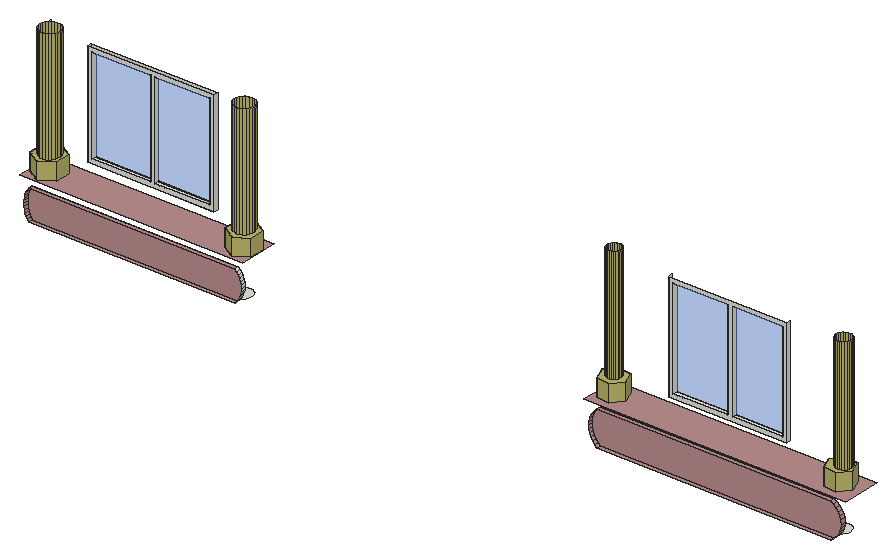
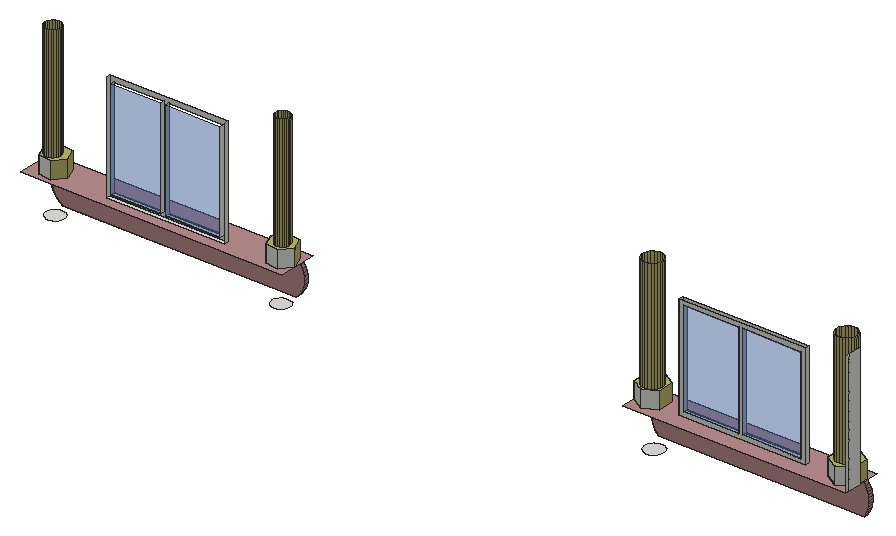
# SketchUp Ruby script. Lengths in inches.
U = 1.inch
M = Sketchup.active_model
def pt(a) = Geom::Point3d.new(a.map { |v| v * U })
def face(e, loops, mat)
  f = e.add_face(loops[0].map { |a| pt(a) })
  loops[1..].each { |l| e.add_face(l.map { |a| pt(a) }).erase! }
  f.material = f.back_material = mat if mat
  f
end
# faces: each face lists its corners as indices into pts; further lists are holes
def faces(e, pts, list, mat = nil) = list.each { |f| face(e, (f[0].is_a?(Array) ? f : [f]).map { |l| l.map { |i| pts[i] } }, mat) }
# xy, xz, yz: faces in a plane at the given z, y or x. An outline is a flat list of corners, or four numbers for a rectangle; further outlines are holes
def ring(l) = l.size == 4 ? [[l[0], l[1]], [l[2], l[1]], [l[2], l[3]], [l[0], l[3]]] : l.each_slice(2).to_a
def flat(e, list, mat, &to3) = list.each { |f| face(e, (f[0].is_a?(Array) ? f : [f]).map { |l| ring(l).map { |u, v| to3.(u, v) } }, mat) }
def xy(e, z, list, mat = nil) = flat(e, list, mat) { |x, y| [x, y, z] }
def xz(e, y, list, mat = nil) = flat(e, list, mat) { |x, z| [x, y, z] }
def yz(e, x, list, mat = nil) = flat(e, list, mat) { |y, z| [x, y, z] }
def lines(e, pts, list) = list.each { |a, b| e.add_line(pt(pts[a]), pt(pts[b])) }
# prism: a flat outline (further loops are holes) pulled along v
def prism(e, loops, v, mat = nil)
  f = face(e, loops, mat); d = Geom::Vector3d.new(v.map { |x| x * U })
  f.pushpull(f.normal.samedirection?(d) ? d.length : -d.length)
end
def box(e, o, s, mat = nil) = prism(e, [[o, [o[0] + s[0], o[1], o[2]], [o[0] + s[0], o[1] + s[1], o[2]], [o[0], o[1] + s[1], o[2]]]], [0, 0, s[2]], mat)
def at(x, y, z, deg = 0) = Geom::Transformation.translation(pt([x, y, z])) * Geom::Transformation.rotation(ORIGIN, Z_AXIS, deg.degrees)
def axes(o, x, y, z) = Geom::Transformation.new([*x, 0, *y, 0, *z, 0, *pt(o).to_a, 1])
def part(name) = M.definitions.add(name)
# library, detail: a bought-in or finely detailed component or shape, given as its bounding box
def library(name, o, s) = part(name).tap { |d| box(d.entities, o, s) }
def detail(e, o, s) = box(e.add_group.entities, o, s)
def put(e, d, t, mat = nil) = e.add_instance(d, t).tap { |i| i.material = mat if mat }
def group(e, t, mat = nil) = e.add_group.tap { |g| g.transformation = t; g.material = mat if mat }.entities
root = M.entities
M.materials.add("[0057_DarkKhaki]").color = [189, 183, 107]
M.materials.add("[0119_RosyBrown]").color = [188, 143, 143]
M.materials.add("[Translucent Glass Blue]").color = [100, 149, 237]
M.materials["[Translucent Glass Blue]"].alpha = 0.5
xy(root,364,[[551.49,97.26,553.12,97.47,554.64,98.1,555.95,99.11,556.95,100.41,557.58,101.9375,557.8,103.57,557.58,105.2,556.95,106.73,555.95,108.03,554.64,109.04,553.12,109.67,551.49,109.88,549.85,109.67,548.33,109.04,547.02,108.03,546.02,106.73,545.39,105.2,545.17,103.57,545.39,101.9375,546.02,100.41,547.02,99.11,548.33,98.1,549.85,97.47],[711.11,97.26,712.74,97.47,714.27,98.1,715.57,99.11,716.58,100.41,717.21,101.9375,717.42,103.57,717.21,105.2,716.58,106.73,715.57,108.03,714.27,109.04,712.74,109.67,711.11,109.88,709.48,109.67,707.95,109.04,706.65,108.03,705.64,106.73,705.01,105.2,704.8,103.57,705.01,101.9375,705.64,100.41,706.65,99.11,707.95,98.1,709.48,97.47]])
xy(root,364,[[549.67,89.37,714.61,92.37]],"[0119_RosyBrown]")
xy(root,364.25,[[287.6,96.4,289.34,96.48,291.01,97.01,292.47,97.96,293.65,99.25,294.45,100.8,294.82,102.51,294.74,104.25,294.21,105.91,293.26,107.38,291.97,108.56,290.42,109.36,288.71,109.73,286.97,109.65,285.31,109.11,283.84,108.17,282.66,106.88,281.86,105.33,281.49,103.62,281.58,101.88,282.11,100.22,283.05,98.75,284.34,97.57,285.89,96.77]])
xy(root,366,[[148.36,89.37,293.68,92.37]],"[0119_RosyBrown]")
xy(root,387.6875,[[148.36,89.37,293.68,92.37]],"[0119_RosyBrown]")
xy(root,388.75,[[549.67,89.37,714.61,92.37]],"[0119_RosyBrown]")
xy(root,391.75,[[540.59,104.78,540.59,105.17,540.49,105.04]])
xy(root,391.75,[[[540.59,89.37,725.37,89.37,725.37,116.37,540.59,116.37,540.59,105.17,546.55,112.6,556.13,111.125,559.64,102.1,553.58,94.54,544,96.01,540.59,104.78],[713.95,94.54,704.38,96.01,700.87,105.04,706.93,112.6,716.5,111.125,720.02,102.1]]],"[0119_RosyBrown]")
xy(root,393.6875,[[152.83,91.15,143.52,96.53,143.52,107.28,152.83,112.65,162.14,107.28,162.14,96.53],[290.08,91.15,280.77,96.53,280.77,107.28,290.08,112.65,299.39,107.28,299.39,96.53]])
xy(root,393.6875,[[[142.36,89.37,299.68,116.37],[290.08,91.15,280.77,96.53,280.77,107.28,290.08,112.65,299.39,107.28,299.39,96.53],[152.83,91.15,143.52,96.53,143.52,107.28,152.83,112.65,162.14,107.28,162.14,96.53]]],"[0119_RosyBrown]")
xy(root,397.08,[[581.28,113.37,664.4,116.37]])
xy(root,400.08,[[584.28,113.37,622.84,116.37],[626.17,113.37,661.4,116.37]])
xy(root,401.45,[[170.78,113.37,260.03,116.37]])
xy(root,403.75,[[711.84,99.06,710.41,99.24,709.09,99.79,707.95,100.67,707.07,101.81,706.53,103.13,706.34,104.56,706.53,105.98,707.07,107.31,707.95,108.44,709.09,109.32,710.41,109.87,711.84,110.06,713.26,109.87,714.59,109.32,715.73,108.44,716.6,107.31,717.15,105.98,717.34,104.56,717.15,103.13,716.6,101.81,715.73,100.67,714.59,99.79,713.26,99.24]])
xy(root,403.75,[[[553.58,94.54,559.64,102.1,556.13,111.125,546.55,112.6,540.59,105.17,540.59,104.78,544,96.01],[549.01,99.72,547.78,100.05,546.67,100.68,545.77,101.58,545.13,102.68,544.8,103.91,544.8,105.19,545.13,106.41,545.76,107.52,546.66,108.42,547.76,109.06,548.99,109.39,550.26,109.39,551.49,109.0625,552.6,108.43,553.5,107.53,554.14,106.43,554.47,105.2,554.47,103.93,554.14,102.7,553.51,101.59,552.61,100.69,551.51,100.05,550.28,99.72]],[[713.95,94.54,720.02,102.1,716.5,111.125,706.93,112.6,700.87,105.04,704.38,96.01],[711.84,99.06,710.41,99.24,709.09,99.79,707.95,100.67,707.07,101.81,706.53,103.13,706.34,104.56,706.53,105.98,707.07,107.31,707.95,108.44,709.09,109.32,710.41,109.87,711.84,110.06,713.26,109.87,714.59,109.32,715.73,108.44,716.6,107.31,717.15,105.98,717.34,104.56,717.15,103.13,716.6,101.81,715.73,100.67,714.59,99.79,713.26,99.24]]],"[0057_DarkKhaki]")
xy(root,404.45,[[173.78,113.37,215.4,116.37],[217.84,113.37,257.03,116.37]])
xy(root,405.6875,[[153.73,94.92,151.91,95.02,150.17,95.59,148.64,96.6,147.43,97.96,146.6,99.59,146.23,101.38,146.33,103.2,146.91,104.94,147.91,106.47,149.27,107.69,150.9,108.51,152.69,108.88,154.52,108.78,156.25,108.21,157.78,107.2,159,105.84,159.82,104.21,160.19,102.42,160.09,100.6,159.52,98.86,158.52,97.33,157.15,96.12,155.52,95.29],[289.98,96.17,288.16,96.27,286.42,96.84,284.89,97.85,283.68,99.21,282.85,100.84,282.48,102.63,282.58,104.45,283.16,106.19,284.16,107.72,285.52,108.94,287.15,109.76,288.94,110.13,290.77,110.03,292.5,109.46,294.03,108.45,295.25,107.09,296.07,105.46,296.44,103.67,296.34,101.85,295.77,100.11,294.77,98.58,293.4,97.37,291.77,96.54]])
xy(root,405.6875,[[[152.83,91.15,162.14,96.53,162.14,107.28,152.83,112.65,143.52,107.28,143.52,96.53],[153.73,94.92,151.91,95.02,150.17,95.59,148.64,96.6,147.43,97.96,146.6,99.59,146.23,101.38,146.33,103.2,146.91,104.94,147.91,106.47,149.27,107.69,150.9,108.51,152.69,108.88,154.52,108.78,156.25,108.21,157.78,107.2,159,105.84,159.82,104.21,160.19,102.42,160.09,100.6,159.52,98.86,158.52,97.33,157.15,96.12,155.52,95.29]],[[290.08,91.15,299.39,96.53,299.39,107.28,290.08,112.65,280.77,107.28,280.77,96.53],[289.98,96.17,288.16,96.27,286.42,96.84,284.89,97.85,283.68,99.21,282.85,100.84,282.48,102.63,282.58,104.45,283.16,106.19,284.16,107.72,285.52,108.94,287.15,109.76,288.94,110.13,290.77,110.03,292.5,109.46,294.03,108.45,295.25,107.09,296.07,105.46,296.44,103.67,296.34,101.85,295.77,100.11,294.77,98.58,293.4,97.37,291.77,96.54]]],"[0057_DarkKhaki]")
xz(root,92.37,[[549.67,364,714.61,364,716.81,365.33,718.71,367.04,720.27,369.07,721.42,371.36,722.13,373.82,722.37,376.375,722.13,378.93,721.42,381.39,720.27,383.68,718.71,385.71,716.81,387.42,714.61,388.75,549.67,388.75,547.9,387.16,546.4,385.32,545.19,383.27,544.3125,381.0625,543.77,378.75,543.59,376.375,543.77,374,544.3125,371.6875,545.19,369.48,546.4,367.43,547.9,365.59],[148.36,366,293.68,366,295.15,367.43,296.41,369.0625,297.41,370.86,298.14,372.78,298.59,374.79,298.74,376.84,298.59,378.9,298.14,380.9,297.41,382.83,296.41,384.625,295.15,386.26,293.68,387.6875,148.36,387.6875,147.34,386.06,146.48,384.33,145.81,382.53,145.32,380.67,145.03,378.77,144.93,376.84,145.03,374.92,145.32,373.02,145.81,371.16,146.48,369.35,147.34,367.63]],"[0119_RosyBrown]")
xz(root,99.72,[[549.01,403.75,550.28,484.5]],"[0057_DarkKhaki]")
xz(root,109.39,[[548.99,403.75,550.26,484.5]],"[0057_DarkKhaki]")
xz(root,113.37,[[[581.28,397.08,664.4,473.26],[584.28,400.08,622.84,470.26],[626.17,400.08,661.4,470.26]],[[170.78,401.45,260.03,475.13],[173.78,404.45,215.4,472.13],[217.84,404.45,257.03,472.13]]])
xz(root,116.37,[[[170.78,401.45,260.03,475.13],[173.78,404.45,215.4,472.13],[217.84,404.45,257.03,472.13]]])
xz(root,116.37,[[584.28,400.08,622.84,470.26],[626.17,400.08,661.4,470.26],[173.78,404.45,215.4,472.13],[217.84,404.45,257.03,472.13]],"[Translucent Glass Blue]")
yz(root,142.36,[[104.37,393.6875,113.37,480],[113.37,393.6875,116.37,480]])
yz(root,143.52,[[96.53,393.6875,107.28,405.6875]],"[0057_DarkKhaki]")
yz(root,162.14,[[96.53,393.6875,107.28,405.6875]],"[0057_DarkKhaki]")
yz(root,170.78,[[113.37,401.45,116.37,475.13]])
yz(root,173.78,[[113.37,404.45,116.37,472.13]])
yz(root,215.4,[[113.37,404.45,116.37,472.13]])
yz(root,217.84,[[113.37,404.45,116.37,472.13]])
yz(root,257.03,[[113.37,404.45,116.37,472.13]])
yz(root,260.03,[[113.37,401.45,116.37,475.13]])
yz(root,280.77,[[96.53,393.6875,107.28,405.6875]],"[0057_DarkKhaki]")
yz(root,299.39,[[96.53,393.6875,107.28,405.6875]],"[0057_DarkKhaki]")
yz(root,540.59,[[104.78,391.75,105.17,403.75]])
yz(root,544.8,[[103.91,403.75,105.19,484.5]],"[0057_DarkKhaki]")
yz(root,554.47,[[103.93,403.75,105.2,484.5]],"[0057_DarkKhaki]")
yz(root,581.28,[[113.37,397.08,116.37,473.26]])
yz(root,584.28,[[113.37,400.08,116.37,470.26]])
yz(root,622.84,[[113.37,400.08,116.37,470.26]])
yz(root,626.17,[[113.37,400.08,116.37,470.26]])
yz(root,661.4,[[113.37,400.08,116.37,470.26]])
yz(root,664.4,[[113.37,397.08,116.37,473.26]])
p = [[549.67,92.37,364],[547.9,92.37,365.59],[547.9,89.37,365.59],[549.67,89.37,364],[716.81,92.37,365.33],[714.61,92.37,364],
  [714.61,89.37,364],[716.81,89.37,365.33],[718.71,92.37,367.04],[718.71,89.37,367.04],[546.4,92.37,367.43],[546.4,89.37,367.43],
  [148.36,92.37,366],[147.34,92.37,367.63],[147.34,89.37,367.63],[148.36,89.37,366],[295.15,92.37,367.43],[293.68,92.37,366],
  [293.68,89.37,366],[295.15,89.37,367.43],[720.27,92.37,369.07],[720.27,89.37,369.07],[296.41,92.37,369.0625],[296.41,89.37,369.0625],
  [545.19,92.37,369.48],[545.19,89.37,369.48],[146.48,92.37,369.35],[146.48,89.37,369.35],[297.41,92.37,370.86],[297.41,89.37,370.86],
  [721.42,92.37,371.36],[721.42,89.37,371.36],[145.81,92.37,371.16],[145.81,89.37,371.16],[544.3125,92.37,371.6875],[544.3125,89.37,371.6875],
  [298.14,92.37,372.78],[298.14,89.37,372.78],[145.32,92.37,373.02],[145.32,89.37,373.02],[722.13,92.37,373.82],[722.13,89.37,373.82],
  [543.77,92.37,374],[543.77,89.37,374],[298.59,92.37,374.79],[298.59,89.37,374.79],[145.03,92.37,374.92],[145.03,89.37,374.92],
  [722.37,92.37,376.375],[722.37,89.37,376.375],[543.59,92.37,376.375],[543.59,89.37,376.375],[298.74,92.37,376.84],[298.74,89.37,376.84],
  [144.93,92.37,376.84],[144.93,89.37,376.84],[543.77,92.37,378.75],[543.77,89.37,378.75],[722.13,92.37,378.93],[722.13,89.37,378.93],
  [145.03,92.37,378.77],[145.03,89.37,378.77],[298.59,92.37,378.9],[298.59,89.37,378.9],[544.3125,92.37,381.0625],[544.3125,89.37,381.0625],
  [145.32,92.37,380.67],[145.32,89.37,380.67],[298.14,92.37,380.9],[298.14,89.37,380.9],[721.42,92.37,381.39],[721.42,89.37,381.39],
  [145.81,92.37,382.53],[145.81,89.37,382.53],[297.41,92.37,382.83],[297.41,89.37,382.83],[545.19,92.37,383.27],[545.19,89.37,383.27],
  [720.27,92.37,383.68],[720.27,89.37,383.68],[146.48,92.37,384.33],[146.48,89.37,384.33],[296.41,92.37,384.625],[296.41,89.37,384.625],
  [546.4,92.37,385.32],[546.4,89.37,385.32],[718.71,92.37,385.71],[718.71,89.37,385.71],[147.34,92.37,386.06],[147.34,89.37,386.06],
  [295.15,92.37,386.26],[295.15,89.37,386.26],[547.9,92.37,387.16],[547.9,89.37,387.16],[716.81,92.37,387.42],[716.81,89.37,387.42],
  [148.36,92.37,387.6875],[148.36,89.37,387.6875],[293.68,92.37,387.6875],[293.68,89.37,387.6875],[549.67,92.37,388.75],[549.67,89.37,388.75],
  [714.61,92.37,388.75],[714.61,89.37,388.75],[544,96.01,391.75],[553.58,94.54,391.75],[553.58,94.54,403.75],[544,96.01,403.75],
  [559.64,102.1,391.75],[559.64,102.1,403.75],[704.38,96.01,391.75],[713.95,94.54,391.75],[713.95,94.54,403.75],[704.38,96.01,403.75],
  [720.02,102.1,391.75],[720.02,102.1,403.75],[540.59,104.78,391.75],[540.59,104.78,403.75],[700.87,105.04,391.75],[700.87,105.04,403.75],
  [556.13,111.125,391.75],[556.13,111.125,403.75],[716.5,111.125,391.75],[716.5,111.125,403.75],[706.93,112.6,391.75],[706.93,112.6,403.75],
  [546.55,112.6,391.75],[540.59,105.17,391.75],[540.59,105.17,403.75],[546.55,112.6,403.75],[143.52,96.53,393.6875],[152.83,91.15,393.6875],
  [152.83,91.15,405.6875],[143.52,96.53,405.6875],[162.14,96.53,393.6875],[162.14,96.53,405.6875],[280.77,96.53,393.6875],[290.08,91.15,393.6875],
  [290.08,91.15,405.6875],[280.77,96.53,405.6875],[299.39,96.53,393.6875],[299.39,96.53,405.6875],[152.83,112.65,393.6875],[143.52,107.28,393.6875],
  [143.52,107.28,405.6875],[152.83,112.65,405.6875],[162.14,107.28,393.6875],[162.14,107.28,405.6875],[290.08,112.65,393.6875],[280.77,107.28,393.6875],
  [280.77,107.28,405.6875],[290.08,112.65,405.6875],[299.39,107.28,393.6875],[299.39,107.28,405.6875],[710.41,99.24,403.75],[711.84,99.06,403.75],
  [711.84,99.06,484.5],[710.41,99.24,484.5],[713.26,99.24,403.75],[713.26,99.24,484.5],[709.09,99.79,403.75],[709.09,99.79,484.5],
  [714.59,99.79,403.75],[714.59,99.79,484.5],[547.78,100.05,403.75],[549.01,99.72,403.75],[549.01,99.72,484.5],[547.78,100.05,484.5],
  [550.28,99.72,403.75],[551.51,100.05,403.75],[551.51,100.05,484.5],[550.28,99.72,484.5],[707.95,100.67,403.75],[707.95,100.67,484.5],
  [715.73,100.67,403.75],[715.73,100.67,484.5],[546.67,100.68,403.75],[546.67,100.68,484.5],[552.61,100.69,403.75],[552.61,100.69,484.5],
  [545.77,101.58,403.75],[545.77,101.58,484.5],[553.51,101.59,403.75],[553.51,101.59,484.5],[707.07,101.81,403.75],[707.07,101.81,484.5],
  [716.6,101.81,403.75],[716.6,101.81,484.5],[545.13,102.68,403.75],[545.13,102.68,484.5],[554.14,102.7,403.75],[554.14,102.7,484.5],
  [706.53,103.13,403.75],[706.53,103.13,484.5],[717.15,103.13,403.75],[717.15,103.13,484.5],[544.8,103.91,403.75],[544.8,103.91,484.5],
  [554.47,103.93,403.75],[554.47,103.93,484.5],[706.34,104.56,403.75],[706.34,104.56,484.5],[717.34,104.56,403.75],[717.34,104.56,484.5],
  [706.53,105.98,403.75],[706.53,105.98,484.5],[717.15,105.98,403.75],[717.15,105.98,484.5],[545.13,106.41,403.75],[544.8,105.19,403.75],
  [544.8,105.19,484.5],[545.13,106.41,484.5],[554.47,105.2,403.75],[554.14,106.43,403.75],[554.14,106.43,484.5],[554.47,105.2,484.5],
  [707.07,107.31,403.75],[707.07,107.31,484.5],[716.6,107.31,403.75],[716.6,107.31,484.5],[545.76,107.52,403.75],[545.76,107.52,484.5],
  [553.5,107.53,403.75],[553.5,107.53,484.5],[707.95,108.44,403.75],[707.95,108.44,484.5],[715.73,108.44,403.75],[715.73,108.44,484.5],
  [546.66,108.42,403.75],[546.66,108.42,484.5],[552.6,108.43,403.75],[552.6,108.43,484.5],[547.76,109.06,403.75],[547.76,109.06,484.5],
  [551.49,109.0625,403.75],[551.49,109.0625,484.5],[709.09,109.32,403.75],[709.09,109.32,484.5],[714.59,109.32,403.75],[714.59,109.32,484.5],
  [548.99,109.39,403.75],[548.99,109.39,484.5],[550.26,109.39,403.75],[550.26,109.39,484.5],[710.41,109.87,403.75],[710.41,109.87,484.5],
  [713.26,109.87,403.75],[713.26,109.87,484.5],[711.84,110.06,403.75],[711.84,110.06,484.5],[151.91,95.02,405.6875],[153.73,94.92,405.6875],
  [153.73,94.92,485.25],[151.91,95.02,485.25],[155.52,95.29,405.6875],[155.52,95.29,485.25],[150.17,95.59,405.6875],[150.17,95.59,485.25],
  [157.15,96.12,405.6875],[157.15,96.12,485.25],[148.64,96.6,405.6875],[148.64,96.6,485.25],[158.52,97.33,405.6875],[158.52,97.33,485.25],
  [288.16,96.27,405.6875],[289.98,96.17,405.6875],[289.98,96.17,485.25],[288.16,96.27,485.25],[291.77,96.54,405.6875],[291.77,96.54,485.25],
  [286.42,96.84,405.6875],[286.42,96.84,485.25],[293.4,97.37,405.6875],[293.4,97.37,485.25],[147.43,97.96,405.6875],[147.43,97.96,485.25],
  [284.89,97.85,405.6875],[284.89,97.85,485.25],[159.52,98.86,405.6875],[159.52,98.86,485.25],[294.77,98.58,405.6875],[294.77,98.58,485.25],
  [283.68,99.21,405.6875],[283.68,99.21,485.25],[146.6,99.59,405.6875],[146.6,99.59,485.25],[295.77,100.11,405.6875],[295.77,100.11,485.25],
  [160.09,100.6,405.6875],[160.09,100.6,485.25],[282.85,100.84,405.6875],[282.85,100.84,485.25],[146.23,101.38,405.6875],[146.23,101.38,485.25],
  [296.34,101.85,405.6875],[296.34,101.85,485.25],[160.19,102.42,405.6875],[160.19,102.42,485.25],[282.48,102.63,405.6875],[282.48,102.63,485.25],
  [146.33,103.2,405.6875],[146.33,103.2,485.25],[296.44,103.67,405.6875],[296.44,103.67,485.25],[159.82,104.21,405.6875],[159.82,104.21,485.25],
  [282.58,104.45,405.6875],[282.58,104.45,485.25],[146.91,104.94,405.6875],[146.91,104.94,485.25],[296.07,105.46,405.6875],[296.07,105.46,485.25],
  [159,105.84,405.6875],[159,105.84,485.25],[283.16,106.19,405.6875],[283.16,106.19,485.25],[147.91,106.47,405.6875],[147.91,106.47,485.25],
  [295.25,107.09,405.6875],[295.25,107.09,485.25],[157.78,107.2,405.6875],[157.78,107.2,485.25],[284.16,107.72,405.6875],[284.16,107.72,485.25],
  [149.27,107.69,405.6875],[149.27,107.69,485.25],[294.03,108.45,405.6875],[294.03,108.45,485.25],[156.25,108.21,405.6875],[156.25,108.21,485.25],
  [150.9,108.51,405.6875],[150.9,108.51,485.25],[285.52,108.94,405.6875],[285.52,108.94,485.25],[154.52,108.78,405.6875],[154.52,108.78,485.25],
  [152.69,108.88,405.6875],[152.69,108.88,485.25],[292.5,109.46,405.6875],[292.5,109.46,485.25],[287.15,109.76,405.6875],[287.15,109.76,485.25],
  [290.77,110.03,405.6875],[290.77,110.03,485.25],[288.94,110.13,405.6875],[288.94,110.13,485.25]]
faces(root,p,[[0,1,2,3],[4,5,6,7],[8,4,7,9],[1,10,11,2],[12,13,14,15],[20,8,9,21],[10,24,25,11],[13,26,27,14],
  [30,20,21,31],[26,32,33,27],[24,34,35,25],[32,38,39,33],[40,30,31,41],[34,42,43,35],[38,46,47,39],[48,40,41,49],
  [42,50,51,43],[46,54,55,47],[50,56,57,51],[58,48,49,59],[54,60,61,55],[56,64,65,57],[60,66,67,61],[70,58,59,71],
  [66,72,73,67],[64,76,77,65],[78,70,71,79],[72,80,81,73],[76,84,85,77],[86,78,79,87],[80,88,89,81],[84,92,93,85],
  [94,86,87,95],[88,96,97,89],[92,100,101,93],[102,94,95,103]],"[0119_RosyBrown]")
faces(root,p,[[16,17,18,19],[22,16,19,23],[28,22,23,29],[36,28,29,37],[44,36,37,45],[52,44,45,53],[62,52,53,63],[68,62,63,69],
  [74,68,69,75],[82,74,75,83],[90,82,83,91],[98,90,91,99],[126,127,128,129],[120,126,129,121],[122,124,125,123],[142,143,144,145],
  [146,142,145,147],[148,149,150,151],[152,148,151,153]])
faces(root,p,[[104,105,106,107],[105,108,109,106],[110,111,112,113],[111,114,115,112],[116,104,107,117],[118,110,113,119],[108,120,121,109],[114,122,123,115],
  [124,118,119,125],[130,131,132,133],[131,134,135,132],[136,137,138,139],[137,140,141,138],[154,155,156,157],[155,158,159,156],[160,154,157,161],
  [158,162,163,159],[164,165,166,167],[168,169,170,171],[172,160,161,173],[162,174,175,163],[176,164,167,177],[169,178,179,170],[180,176,177,181],
  [178,182,183,179],[184,172,173,185],[174,186,187,175],[188,180,181,189],[182,190,191,183],[192,184,185,193],[186,194,195,187],[196,188,189,197],
  [190,198,199,191],[200,192,193,201],[194,202,203,195],[204,200,201,205],[202,206,207,203],[208,209,210,211],[212,213,214,215],[216,204,205,217],
  [206,218,219,207],[220,208,211,221],[213,222,223,214],[224,216,217,225],[218,226,227,219],[228,220,221,229],[222,230,231,223],[232,228,229,233],
  [230,234,235,231],[236,224,225,237],[226,238,239,227],[240,232,233,241],[234,242,243,235],[244,236,237,245],[238,246,247,239],[248,244,245,249],
  [246,248,249,247],[250,251,252,253],[251,254,255,252],[256,250,253,257],[254,258,259,255],[260,256,257,261],[258,262,263,259],[264,265,266,267],
  [265,268,269,266],[270,264,267,271],[268,272,273,269],[274,260,261,275],[276,270,271,277],[262,278,279,263],[272,280,281,273],[282,276,277,283],
  [284,274,275,285],[280,286,287,281],[278,288,289,279],[290,282,283,291],[292,284,285,293],[286,294,295,287],[288,296,297,289],[298,290,291,299],
  [300,292,293,301],[294,302,303,295],[296,304,305,297],[306,298,299,307],[308,300,301,309],[302,310,311,303],[304,312,313,305],[314,306,307,315],
  [316,308,309,317],[310,318,319,311],[312,320,321,313],[322,314,315,323],[324,316,317,325],[318,326,327,319],[320,328,329,321],[330,324,325,331],
  [332,322,323,333],[328,334,335,329],[336,330,331,337],[326,338,339,327],[334,336,337,335],[340,332,333,341],[338,342,343,339],[344,340,341,345],
  [342,344,345,343]],"[0057_DarkKhaki]")
